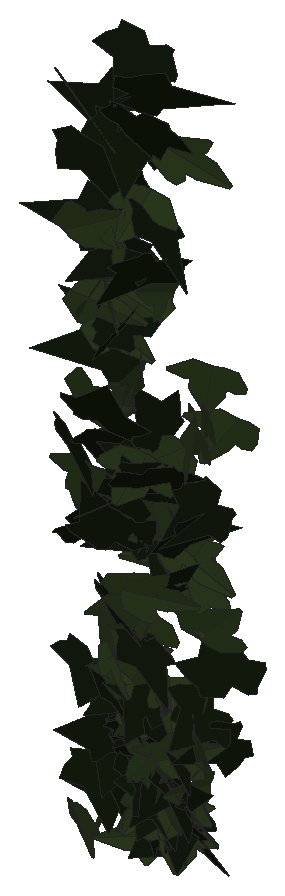
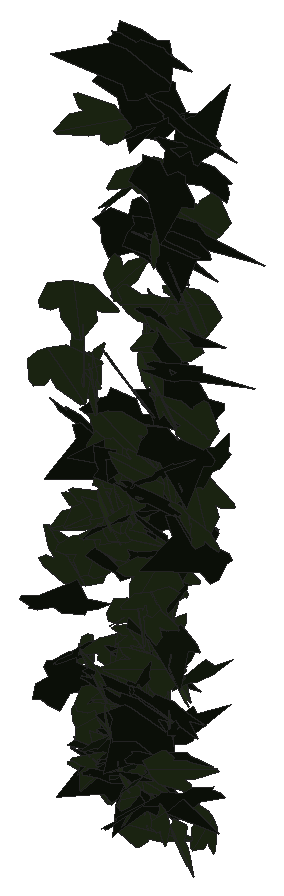
# SketchUp Ruby script. Lengths in inches.
U = 1.inch
M = Sketchup.active_model
def pt(a) = Geom::Point3d.new(a.map { |v| v * U })
def face(e, loops, mat)
  f = e.add_face(loops[0].map { |a| pt(a) })
  loops[1..].each { |l| e.add_face(l.map { |a| pt(a) }).erase! }
  f.material = f.back_material = mat if mat
  f
end
# faces: each face lists its corners as indices into pts; further lists are holes
def faces(e, pts, list, mat = nil) = list.each { |f| face(e, (f[0].is_a?(Array) ? f : [f]).map { |l| l.map { |i| pts[i] } }, mat) }
# xy, xz, yz: faces in a plane at the given z, y or x. An outline is a flat list of corners, or four numbers for a rectangle; further outlines are holes
def ring(l) = l.size == 4 ? [[l[0], l[1]], [l[2], l[1]], [l[2], l[3]], [l[0], l[3]]] : l.each_slice(2).to_a
def flat(e, list, mat, &to3) = list.each { |f| face(e, (f[0].is_a?(Array) ? f : [f]).map { |l| ring(l).map { |u, v| to3.(u, v) } }, mat) }
def xy(e, z, list, mat = nil) = flat(e, list, mat) { |x, y| [x, y, z] }
def xz(e, y, list, mat = nil) = flat(e, list, mat) { |x, z| [x, y, z] }
def yz(e, x, list, mat = nil) = flat(e, list, mat) { |y, z| [x, y, z] }
def lines(e, pts, list) = list.each { |a, b| e.add_line(pt(pts[a]), pt(pts[b])) }
# prism: a flat outline (further loops are holes) pulled along v
def prism(e, loops, v, mat = nil)
  f = face(e, loops, mat); d = Geom::Vector3d.new(v.map { |x| x * U })
  f.pushpull(f.normal.samedirection?(d) ? d.length : -d.length)
end
def box(e, o, s, mat = nil) = prism(e, [[o, [o[0] + s[0], o[1], o[2]], [o[0] + s[0], o[1] + s[1], o[2]], [o[0], o[1] + s[1], o[2]]]], [0, 0, s[2]], mat)
def at(x, y, z, deg = 0) = Geom::Transformation.translation(pt([x, y, z])) * Geom::Transformation.rotation(ORIGIN, Z_AXIS, deg.degrees)
def axes(o, x, y, z) = Geom::Transformation.new([*x, 0, *y, 0, *z, 0, *pt(o).to_a, 1])
def part(name) = M.definitions.add(name)
# library, detail: a bought-in or finely detailed component or shape, given as its bounding box
def library(name, o, s) = part(name).tap { |d| box(d.entities, o, s) }
def detail(e, o, s) = box(e.add_group.entities, o, s)
def put(e, d, t, mat = nil) = e.add_instance(d, t).tap { |i| i.material = mat if mat }
def group(e, t, mat = nil) = e.add_group.tap { |g| g.transformation = t; g.material = mat if mat }.entities
root = M.entities
M.materials.add("1026 AP 7946 SUNNY SIDE UP").color = [254, 231, 186]
M.materials.add("efeu1").color = [18, 25, 13]
M.materials.add("efeu2").color = [43, 57, 29]
c1 = part("ivyleaf_9")
p = [[1.54,2.16,1.25],[1.36,2.04,1.19],[-0.21,0.99,0.68],[-0.71,1.11,0.82],[-0.85,0.86,0.67],[-0.8,0.17,0.21],
  [-0.9,-0.01,0.1],[-0.67,-0.16,-0.02],[-0.08,-0.08,-0.05],[-0.03,-0.6,-0.4],[0.65,-0.88,-0.66],[0.83,-0.6,-0.49],
  [1.29,-0.42,-0.43],[1.8125,-0.07,-0.26],[1.21,0.44,0.15]]
faces(c1.entities,p,[[0,1,2,3,4,5,6,7,8,9,10,11,12,13,14]],"efeu1")
c2 = part("ivyleaf_10")
p = [[0,0.5,-0.03],[-0.0625,2.02,-0.43],[-0.19,2.01,-0.46],[-0.54,1.05,-0.29],[-0.52,0.625,-0.18],[-0.83,0.76,-0.28],
  [-1.16,0.64,-0.33],[-1.15,0.33,-0.24],[-0.77,-0.39,0.02],[-0.3,-0.51,0.16],[0.04,-0.48,0.23],[-0.02,2.01,-0.4375],
  [-0.06,2.01,-0.43],[0.04,-0.49,0.23],[0.67,-0.49,0.14],[1.38,0.36,-0.2],[1.375,0.51,-0.24],[0.81,0.65,-0.19],
  [0.62,0.59,-0.15],[0.6,1.09,-0.28],[0.5,1.23,-0.31]]
faces(c2.entities,p,[[0,1,2,3,4,5,6,7,8,9,10],[11,12,0,13,14,15,16,17,18,19,20]],"efeu2")
put(root,c1,axes([98.49,212.05,269.27],[-0.08526,-0.04089,0.25028],[-0.26767,-0.17357,-0.07103],[0.3023,-0.16522,0.00769]),"1026 AP 7946 SUNNY SIDE UP")
put(root,c1,axes([100.3125,211.96,273.27],[-0.47462,0.04512,-0.05872],[0.08454,-0.03757,-0.30217],[-0.08703,-0.28255,0.02669]),"1026 AP 7946 SUNNY SIDE UP")
put(root,c2,axes([98.93,211.88,271.4375],[-0.2486,-0.25286,-0.0266],[0.04267,0.01175,-0.30667],[0.39716,-0.15954,0.01629]),"1026 AP 7946 SUNNY SIDE UP")
put(root,c1,axes([99.36,211.9375,276.48],[-0.04328,0.20351,-0.24683],[-0.03325,-0.23459,-0.22015],[-0.52438,-0.00192,0.03433]),"1026 AP 7946 SUNNY SIDE UP")
put(root,c2,axes([99.89,212.03,274.12],[0.10442,-0.20831,0.1915],[0.18187,-0.15468,-0.22064],[0.40092,0.12442,0.05022]),"1026 AP 7946 SUNNY SIDE UP")
put(root,c2,axes([99.3,211.71,271.73],[0.1188,0.01973,0.29825],[0.22158,0.2513,-0.0507],[-0.41863,0.13861,0.0578]),"1026 AP 7946 SUNNY SIDE UP")
put(root,c1,axes([98.45,211.95,273.89],[0.44562,-0.02701,0.07349],[-0.11047,0.03739,0.28126],[-0.06013,-0.26883,0.02787]),"1026 AP 7946 SUNNY SIDE UP")
put(root,c1,axes([99.13,211.98,270.85],[0.05244,-0.25972,-0.0269],[0.02039,0.02328,-0.27925],[0.44195,0.02974,0.01607]),"1026 AP 7946 SUNNY SIDE UP")
put(root,c1,axes([97.94,212.08,273.33],[0.07608,-0.21092,0.18856],[0.05391,-0.17609,-0.23326],[0.46636,0.05477,-0.0038]),"1026 AP 7946 SUNNY SIDE UP")
put(root,c2,axes([98.71,211.83,271.2],[-0.01528,0.28786,0.0357],[-0.0625,0.02823,-0.30555],[-0.48723,-0.01265,0.03807]),"1026 AP 7946 SUNNY SIDE UP")
put(root,c1,axes([98.55,211.97,270.13],[0.21081,-0.23004,0.01294],[-0.00284,-0.01803,-0.27991],[0.39132,0.12379,-0.009]),"1026 AP 7946 SUNNY SIDE UP")
put(root,c2,axes([99.02,211.97,270.36],[-0.31309,-0.16797,0.12113],[-0.10904,-0.0997,-0.26681],[0.32824,-0.19334,0.0269]),"1026 AP 7946 SUNNY SIDE UP")
put(root,c2,axes([98.27,211.8,276.67],[-0.19468,-0.13502,0.25878],[0.27493,0.18184,0.19216],[-0.38443,0.19842,0.00638]),"1026 AP 7946 SUNNY SIDE UP")
put(root,c1,axes([99.54,212,269.01],[-0.39901,-0.00249,-0.0961],[0.15113,-0.03869,-0.24905],[-0.01952,-0.2486,0.03617]),"1026 AP 7946 SUNNY SIDE UP")
put(root,c2,axes([98.78,211.89,270.68],[0.12003,0.27677,0.00795],[0.02085,0.0008,-0.30555],[-0.46941,0.0708,-0.01154]),"1026 AP 7946 SUNNY SIDE UP")
put(root,c1,axes([98.2,212.13,270.18],[-0.14201,-0.2201,0.15342],[0.0431,-0.1654,-0.23372],[0.41674,-0.0579,0.07645]),"1026 AP 7946 SUNNY SIDE UP")
put(root,c1,axes([99.3125,212.05,270.1875],[-0.33829,-0.16192,-0.01215],[0.02958,-0.00682,-0.27444],[0.27371,-0.19938,0.01464]),"1026 AP 7946 SUNNY SIDE UP")
put(root,c2,axes([99.08,211.98,273.4375],[0.45671,0.01173,-0.07246],[-0.10874,-0.02673,-0.29867],[-0.02776,0.29767,-0.0222]),"1026 AP 7946 SUNNY SIDE UP")
put(root,c1,axes([99.35,211.76,273.47],[0.33646,0.22451,0.00758],[0.00453,0.00318,-0.32058],[-0.38116,0.19822,0.00287]),"1026 AP 7946 SUNNY SIDE UP")
put(root,c1,axes([99.52,212.02,268.78],[0.01263,0.02538,0.27384],[0.21354,-0.22314,0.0167],[0.37988,0.12459,-0.01849]),"1026 AP 7946 SUNNY SIDE UP")
put(root,c1,axes([99.57,212.11,268.89],[0.01837,-0.23873,0.13227],[0.04929,-0.12501,-0.25663],[0.4561,0.02313,0.0224]),"1026 AP 7946 SUNNY SIDE UP")
put(root,c2,axes([99.14,212.03,277.28],[0.27821,0.18123,-0.16405],[-0.15931,-0.12467,-0.26303],[-0.37287,0.18849,-0.01002]),"1026 AP 7946 SUNNY SIDE UP")
put(root,c2,axes([99.23,211.9375,269.24],[0.26332,-0.18194,-0.08992],[-0.10371,0.05507,-0.25496],[0.32223,0.1664,-0.00858]),"1026 AP 7946 SUNNY SIDE UP")
put(root,c2,axes([99.97,212.16,268.96],[-0.03352,-0.02334,-0.29645],[-0.17499,-0.26543,0.02913],[-0.41865,0.11282,0.01156]),"1026 AP 7946 SUNNY SIDE UP")
put(root,c1,axes([98.6875,211.99,272.21],[0.28824,0.02675,0.2393],[-0.36625,0.04462,0.18444],[-0.02952,-0.2924,0.04828]),"1026 AP 7946 SUNNY SIDE UP")
put(root,c2,axes([99.37,212.02,268.76],[-0.19495,0.11913,-0.18588],[0.18776,-0.13624,-0.17871],[-0.30673,-0.15911,0.00875]),"1026 AP 7946 SUNNY SIDE UP")
put(root,c2,axes([98.11,211.96,268.04],[-0.29628,0.16092,-0.07796],[0.06673,-0.06741,-0.25401],[-0.29383,-0.17757,0.02092]),"1026 AP 7946 SUNNY SIDE UP")
put(root,c1,axes([98.77,212.11,278.14],[-0.13359,-0.27269,0.00935],[0.00737,-0.01404,-0.30392],[0.46331,-0.0784,0.00753]),"1026 AP 7946 SUNNY SIDE UP")
put(root,c1,axes([98.75,211.8,272.84],[0.02401,0.27249,0.04118],[-0.06208,0.03651,-0.28875],[-0.4622,0.00925,0.04092]),"1026 AP 7946 SUNNY SIDE UP")
put(root,c1,axes([98.54,211.96,271.42],[0.33692,-0.191,-0.08782],[-0.1101,0.04723,-0.29401],[0.33351,0.20854,-0.00835]),"1026 AP 7946 SUNNY SIDE UP")
put(root,c2,axes([100.11,211.86,269.88],[-0.24734,0.19341,0.15786],[-0.20793,0.08679,-0.25463],[-0.35368,-0.18628,0.0393]),"1026 AP 7946 SUNNY SIDE UP")
put(root,c2,axes([99.74,211.82,269.4375],[-0.10782,-0.08442,0.26473],[0.17577,0.22674,0.11402],[-0.40917,0.11965,-0.02078]),"1026 AP 7946 SUNNY SIDE UP")
put(root,c2,axes([99.53,212.11,269.21],[0.08542,-0.22565,0.13653],[0.0635,-0.12783,-0.23971],[0.40759,0.0672,0.00873]),"1026 AP 7946 SUNNY SIDE UP")
put(root,c2,axes([99.66,212.03,268.72],[0.42575,0.02925,-0.03108],[-0.04494,-0.02593,-0.26961],[-0.05421,0.25119,-0.02062]),"1026 AP 7946 SUNNY SIDE UP")
put(root,c1,axes([99.11,211.9,278.52],[0.44169,0.07275,-0.14611],[-0.21125,-0.06319,-0.28894],[-0.15825,0.28739,-0.02208]),"1026 AP 7946 SUNNY SIDE UP")
put(root,c1,axes([99.44,212.12,269.72],[0.07739,-0.27307,0.04078],[0.00434,-0.04179,-0.29694],[0.46889,0.04546,-0.00398]),"1026 AP 7946 SUNNY SIDE UP")
put(root,c1,axes([99.54,212.0625,268.88],[0.28147,-0.18304,0.0415],[0.02674,-0.04115,-0.26444],[0.31735,0.16581,-0.01453]),"1026 AP 7946 SUNNY SIDE UP")
put(root,c1,axes([99.9,211.75,272.81],[-0.06446,0.12816,-0.2886],[-0.07842,0.27686,0.13926],[0.47906,0.06257,-0.01603]),"1026 AP 7946 SUNNY SIDE UP")
put(root,c2,axes([99.67,212.03,269.39],[-0.3948,-0.1276,0.05685],[-0.06168,-0.04718,-0.28355],[0.22751,-0.23423,0.02177]),"1026 AP 7946 SUNNY SIDE UP")
put(root,c1,axes([99.21,212.1,277.07],[0.14985,-0.28792,-0.01824],[-0.02233,0.00986,-0.32209],[0.48876,0.08872,-0.00912]),"1026 AP 7946 SUNNY SIDE UP")
put(root,c1,axes([99.11,212.13,270.1875],[-0.41299,-0.06368,0.05582],[-0.07815,-0.03269,-0.26887],[0.1169,-0.24683,0.01747]),"1026 AP 7946 SUNNY SIDE UP")
put(root,c2,axes([99.14,211.9,274.875],[0.11185,-0.22747,-0.19349],[-0.00979,0.19069,-0.2409],[0.46244,0.05905,0.0417]),"1026 AP 7946 SUNNY SIDE UP")
put(root,c1,axes([99.29,212.1875,268.67],[-0.24745,-0.19467,0.04233],[0.01274,-0.05747,-0.25764],[0.33785,-0.14041,0.04072]),"1026 AP 7946 SUNNY SIDE UP")
put(root,c1,axes([98.16,212.09,277.78],[-0.18749,-0.08809,-0.27062],[0.41068,0.08134,-0.14303],[0.19018,-0.26249,0.04207]),"1026 AP 7946 SUNNY SIDE UP")
put(root,c2,axes([98.23,211.97,275.6],[-0.18093,-0.06005,-0.26458],[0.41406,0.04874,-0.12502],[0.11762,-0.26396,0.03311]),"1026 AP 7946 SUNNY SIDE UP")
put(root,c2,axes([99.35,212.01,270.26],[-0.19379,0.23095,-0.0201],[-0.00312,-0.02518,-0.27582],[-0.39377,-0.11346,0.01208]),"1026 AP 7946 SUNNY SIDE UP")
put(root,c2,axes([99.6,212.0625,268.3125],[0.43887,0.08135,0.03336],[0.06002,-0.01243,-0.28934],[-0.13446,0.25998,-0.02028]),"1026 AP 7946 SUNNY SIDE UP")
put(root,c1,axes([98.84,212.14,276.41],[-0.44653,-0.01259,0.02582],[-0.0384,-0.03178,-0.28048],[0.0261,-0.26224,0.02903]),"1026 AP 7946 SUNNY SIDE UP")
put(root,c2,axes([98.94,212.08,270.25],[0.41497,0.08216,-0.01405],[-0.00863,-0.02919,-0.27509],[-0.14127,0.24312,-0.02445]),"1026 AP 7946 SUNNY SIDE UP")
put(root,c2,axes([100.2,212.06,275.12],[-0.41251,-0.12101,0.03925],[-0.03233,-0.04737,-0.29582],[0.19717,-0.26093,0.0336]),"1026 AP 7946 SUNNY SIDE UP")
put(root,c1,axes([99.22,212.09,272.78],[0.24643,0.08014,0.23446],[-0.38294,-0.01237,0.16555],[0.09361,-0.26159,0.06]),"1026 AP 7946 SUNNY SIDE UP")
put(root,c1,axes([99.64,212.01,268.89],[0.34698,-0.11678,-0.10798],[-0.16976,0.02394,-0.25008],[0.19728,0.226,-0.02528]),"1026 AP 7946 SUNNY SIDE UP")
put(root,c2,axes([99.53,212.07,270.28],[0.18975,0.24659,-0.05557],[-0.00721,-0.05843,-0.28989],[-0.42887,0.11008,-0.01971]),"1026 AP 7946 SUNNY SIDE UP")
put(root,c1,axes([99.22,212.02,271.58],[0.31537,0.19631,0.03215],[-0.05859,-0.00504,0.28837],[0.33135,-0.18773,0.02039]),"1026 AP 7946 SUNNY SIDE UP")
put(root,c2,axes([98.67,212.2,276.57],[-0.00223,-0.25766,0.16923],[0.1735,-0.15504,-0.24825],[0.44939,0.05858,0.09668]),"1026 AP 7946 SUNNY SIDE UP")
put(root,c1,axes([98.96,211.9,273.22],[0.07735,0.05221,-0.30263],[0.16453,0.26738,0.07316],[0.46061,-0.10428,0.02469]),"1026 AP 7946 SUNNY SIDE UP")
put(root,c1,axes([99.32,212.13,268.66],[0.02556,-0.26391,-0.0804],[-0.01808,0.07115,-0.28192],[0.46387,0.01731,-0.00656]),"1026 AP 7946 SUNNY SIDE UP")
put(root,c2,axes([98.25,212.0625,272.97],[-0.47545,0.00098,0.09994],[-0.15759,-0.03354,-0.29834],[0.01643,-0.29331,0.0303]),"1026 AP 7946 SUNNY SIDE UP")
put(root,c1,axes([98.87,211.91,270.69],[0.02386,0.28264,0.04639],[-0.07026,0.0413,-0.29887],[-0.47937,0.00801,0.04612]),"1026 AP 7946 SUNNY SIDE UP")
put(root,c1,axes([99.98,212.31,270.03],[-0.19514,-0.20612,0.16734],[-0.10483,-0.15036,-0.24812],[0.40028,-0.13986,0.0166]),"1026 AP 7946 SUNNY SIDE UP")
put(root,c2,axes([98.52,212.09,275.77],[-0.08664,0.25394,-0.05518],[0.00645,-0.05516,-0.27797],[-0.44097,-0.0507,0.00677]),"1026 AP 7946 SUNNY SIDE UP")
put(root,c1,axes([98.48,212.09,276.67],[-0.30459,0.08576,0.20225],[-0.31719,0.03835,-0.20934],[-0.14904,-0.25689,0.0322]),"1026 AP 7946 SUNNY SIDE UP")
put(root,c1,axes([98.15,212.19,278.04],[0.24113,-0.26065,0.08242],[-0.03504,0.08011,0.31822],[-0.4617,-0.14221,0.0189]),"1026 AP 7946 SUNNY SIDE UP")
put(root,c2,axes([98.21,212.11,275.38],[-0.04328,-0.26983,0.00694],[0.01798,0.00904,0.2901],[-0.458,0.02585,0.01073]),"1026 AP 7946 SUNNY SIDE UP")
put(root,c1,axes([99.57,212.24,268.47],[-0.30472,-0.11647,-0.17771],[0.32615,-0.03237,-0.2004],[0.10334,-0.2413,0.10845]),"1026 AP 7946 SUNNY SIDE UP")
put(root,c2,axes([98.39,212.23,270.24],[0.19197,-0.19946,0.14498],[0.09895,-0.12548,-0.24701],[0.39969,0.12687,-0.00849]),"1026 AP 7946 SUNNY SIDE UP")
put(root,c1,axes([98.45,212.1,274.88],[0.10949,0.22576,0.13438],[-0.08997,-0.11197,0.24907],[0.42671,-0.08154,0.01804]),"1026 AP 7946 SUNNY SIDE UP")
put(root,c1,axes([99,211.96,278.8125],[0.29194,0.0355,0.27226],[0.41689,0.06472,-0.18691],[-0.12461,0.29971,0.01255]),"1026 AP 7946 SUNNY SIDE UP")
put(root,c1,axes([99.54,212.11,268.41],[0.42207,-0.08576,-0.0056],[-0.0199,-0.02142,-0.28069],[0.14438,0.24774,-0.0223]),"1026 AP 7946 SUNNY SIDE UP")
put(root,c2,axes([99.23,212.11,272.77],[-0.39394,-0.12203,-0.03602],[0.05942,0.00055,-0.28661],[0.19023,-0.25287,0.01494]),"1026 AP 7946 SUNNY SIDE UP")
put(root,c2,axes([99.16,212.3,268.72],[0.05841,-0.19152,0.2037],[0.10486,-0.18844,-0.20094],[0.42122,0.07347,0.02178]),"1026 AP 7946 SUNNY SIDE UP")
put(root,c2,axes([98.9,212.2,274.65],[0.05826,-0.25237,0.04869],[0.00076,-0.04915,-0.27328],[0.43634,0.03378,-0.00603]),"1026 AP 7946 SUNNY SIDE UP")
put(root,c2,axes([98.7,212.02,269.875],[-0.1634,0.15587,0.17613],[-0.20804,0.11197,-0.19116],[-0.32065,-0.15208,0.03427]),"1026 AP 7946 SUNNY SIDE UP")
put(root,c1,axes([99.46,211.94,274.0625],[-0.0546,0.16525,0.26263],[-0.1632,0.23371,-0.1699],[-0.44765,-0.10536,0.02991]),"1026 AP 7946 SUNNY SIDE UP")
put(root,c1,axes([98.63,212.08,276.54],[0.30356,0.11456,-0.17944],[-0.23576,-0.0966,-0.22864],[-0.25423,0.22637,-0.00222]),"1026 AP 7946 SUNNY SIDE UP")
put(root,c2,axes([98.96,212.05,270.56],[0.16664,0.19262,0.15119],[0.12001,0.11956,-0.22965],[-0.38465,0.12075,-0.00615]),"1026 AP 7946 SUNNY SIDE UP")
put(root,c2,axes([99.12,212.15,270.1875],[-0.40072,0.09197,0.04885],[-0.10835,-0.04549,-0.2629],[-0.13536,-0.23585,0.06583]),"1026 AP 7946 SUNNY SIDE UP")
put(root,c2,axes([98.99,212.27,268.38],[0.13723,0.14304,-0.19504],[-0.17313,-0.15346,-0.17779],[-0.35581,0.12984,0.01128]),"1026 AP 7946 SUNNY SIDE UP")
put(root,c2,axes([98.95,212.26,268.4],[0.16258,0.16533,-0.16092],[-0.1066,-0.13946,-0.20608],[-0.36658,0.11388,-0.01144]),"1026 AP 7946 SUNNY SIDE UP")
put(root,c2,axes([98.96,212.17,269.22],[-0.42744,-0.02083,0.07272],[0.11088,0.03298,0.26945],[-0.04853,0.25878,-0.02479]),"1026 AP 7946 SUNNY SIDE UP")
put(root,c2,axes([100.09,212.07,274.53],[-0.23764,0.20492,0.14312],[-0.19822,0.07485,-0.25674],[-0.33385,-0.19031,0.05056]),"1026 AP 7946 SUNNY SIDE UP")
put(root,c2,axes([99.36,212.17,273.27],[-0.43994,-0.01915,0.04062],[-0.05752,-0.03955,-0.28667],[0.03824,-0.27979,0.03606]),"1026 AP 7946 SUNNY SIDE UP")
put(root,c2,axes([98.8125,212.14,271.57],[-0.35546,-0.10517,-0.09093],[0.14305,0.01768,-0.24963],[0.17757,-0.22476,0.01907]),"1026 AP 7946 SUNNY SIDE UP")
put(root,c1,axes([99.3,212.05,267.97],[0.04411,-0.02278,0.26282],[-0.10737,0.23829,0.03413],[-0.40504,-0.06565,0.01958]),"1026 AP 7946 SUNNY SIDE UP")
put(root,c2,axes([98.67,212.19,273.18],[-0.38397,0.15901,0.03637],[-0.1385,-0.06427,-0.27734],[-0.23792,-0.2192,0.10276]),"1026 AP 7946 SUNNY SIDE UP")
put(root,c2,axes([98,212.21,273.94],[-0.17344,0.00845,0.27623],[0.43778,0.01307,0.1091],[-0.01537,0.2771,-0.00969]),"1026 AP 7946 SUNNY SIDE UP")
put(root,c1,axes([98.95,212.3,279.32],[-0.42491,-0.08185,-0.08873],[0.14267,0.00547,-0.28105],[0.13507,-0.26328,0.01771]),"1026 AP 7946 SUNNY SIDE UP")
put(root,c2,axes([99.95,212.09,274.18],[-0.26267,0.1698,0.1675],[-0.23423,0.07637,-0.2408],[-0.28463,-0.21954,0.04358]),"1026 AP 7946 SUNNY SIDE UP")
put(root,c1,axes([98.91,212.37,270.03],[-0.03265,-0.05735,0.24903],[0.03995,-0.23343,-0.06259],[0.40596,0.01836,0.02619]),"1026 AP 7946 SUNNY SIDE UP")
put(root,c2,axes([98.97,212.3,267.85],[0.12192,0.00357,-0.24605],[-0.35232,-0.10259,-0.07256],[-0.16788,0.21789,-0.02641]),"1026 AP 7946 SUNNY SIDE UP")
put(root,c2,axes([99.58,212.125,268.5],[0.16603,0.21283,0.11649],[0.10436,0.08813,-0.24884],[-0.38993,0.11421,-0.017]),"1026 AP 7946 SUNNY SIDE UP")
put(root,c1,axes([99.1,212.25,268.8125],[0.26415,-0.18729,0.04655],[0.08053,-0.02002,-0.25977],[0.31728,0.16101,0.02718]),"1026 AP 7946 SUNNY SIDE UP")
put(root,c1,axes([98.99,212.25,272.32],[-0.38519,0.09361,0.03807],[-0.07129,-0.01231,-0.26134],[-0.15351,-0.22916,0.02585]),"1026 AP 7946 SUNNY SIDE UP")
put(root,c1,axes([98.875,212.22,268.43],[-0.11281,0.00389,-0.26879],[-0.38799,-0.10861,0.06144],[-0.17673,0.23597,0.0367]),"1026 AP 7946 SUNNY SIDE UP")
put(root,c1,axes([98,212.03,272.17],[0.27391,0.14899,0.18303],[0.24319,0.09261,-0.23253],[-0.2952,0.21454,-0.02173]),"1026 AP 7946 SUNNY SIDE UP")
put(root,c2,axes([98.92,212.14,269.71],[0.15026,0.08253,0.253],[0.33257,0.13135,-0.12642],[-0.26172,0.21429,-0.01539]),"1026 AP 7946 SUNNY SIDE UP")
put(root,c1,axes([100.26,212.44,269.64],[-0.08847,-0.06742,-0.26859],[0.09099,-0.26277,0.05569],[-0.41295,-0.04345,0.06981]),"1026 AP 7946 SUNNY SIDE UP")
put(root,c1,axes([98.78,212.18,275.17],[-0.11859,0.10059,0.25021],[-0.36171,0.10694,-0.11663],[-0.23232,-0.21785,0.05387]),"1026 AP 7946 SUNNY SIDE UP")
put(root,c1,axes([99.17,212.43,267.93],[-0.16818,-0.1416,0.17778],[-0.10889,-0.15752,-0.18493],[0.35661,-0.11488,0.02738]),"1026 AP 7946 SUNNY SIDE UP")
put(root,c1,axes([98.21,212.34,268.59],[-0.1389,-0.25209,-0.07059],[0.04143,0.06185,-0.27479],[0.40809,-0.09208,0.00387]),"1026 AP 7946 SUNNY SIDE UP")
put(root,c1,axes([98.75,212.4,268.73],[0.02971,-0.24978,0.08462],[0.01307,-0.08317,-0.25853],[0.41394,0.02055,0.00209]),"1026 AP 7946 SUNNY SIDE UP")
put(root,c2,axes([99.2,212.43,275.79],[-0.05226,-0.07479,-0.26571],[-0.15187,-0.23046,0.08336],[-0.4113,0.0946,0.00298]),"1026 AP 7946 SUNNY SIDE UP")
put(root,c1,axes([98.56,212.16,278.33],[-0.22742,0.14869,0.20285],[-0.25248,0.11665,-0.21114],[-0.31829,-0.19877,0.02255]),"1026 AP 7946 SUNNY SIDE UP")
put(root,c1,axes([98.98,212.19,268.43],[0.40217,-0.0539,-0.12581],[-0.20256,-0.00057,-0.25882],[0.08163,0.26415,-0.02239]),"1026 AP 7946 SUNNY SIDE UP")
put(root,c1,axes([98.5,212.38,274.74],[-0.39094,0.00094,0.18538],[-0.27903,-0.09178,-0.2348],[0.09241,-0.27312,0.0753]),"1026 AP 7946 SUNNY SIDE UP")
put(root,c2,axes([99.99,212.23,271.18],[-0.38583,-0.06835,0.14576],[0.20126,0.06647,0.26143],[-0.14426,0.27553,-0.02511]),"1026 AP 7946 SUNNY SIDE UP")
put(root,c2,axes([99.64,212.31,271.6875],[-0.43755,-0.10065,-0.04351],[0.13154,-0.10125,-0.26769],[0.12786,-0.24028,0.12648]),"1026 AP 7946 SUNNY SIDE UP")
put(root,c2,axes([98.34,212.18,275.13],[0.20342,0.09152,0.23278],[0.32311,0.10431,-0.15873],[-0.23343,0.22414,-0.01685]),"1026 AP 7946 SUNNY SIDE UP")
put(root,c2,axes([98.98,212.27,270.99],[-0.43322,-0.02522,0.06308],[-0.0865,-0.06897,-0.26736],[0.06683,-0.25275,0.06284]),"1026 AP 7946 SUNNY SIDE UP")
put(root,c1,axes([98.41,212.16,273.6],[0.13483,0.23646,-0.07195],[-0.03586,-0.06705,-0.26798],[-0.41722,0.08218,-0.00022]),"1026 AP 7946 SUNNY SIDE UP")
put(root,c2,axes([99.38,212.28,273.61],[0.36263,-0.04286,-0.18137],[-0.28413,0.02358,-0.23278],[0.08199,0.27127,-0.00452]),"1026 AP 7946 SUNNY SIDE UP")
put(root,c2,axes([98.76,212.32,273.04],[-0.00344,-0.02062,-0.2807],[0.40137,-0.11437,0.00608],[-0.1945,-0.23565,0.01752]),"1026 AP 7946 SUNNY SIDE UP")
put(root,c2,axes([100.27,212.36,274.25],[-0.33215,-0.16514,0.14756],[-0.1184,-0.13338,-0.27182],[0.32372,-0.21822,0.05198]),"1026 AP 7946 SUNNY SIDE UP")
put(root,c1,axes([99.6,212.32,269.77],[-0.37624,0.0542,0.11932],[-0.19204,0.0012,-0.243],[-0.08323,-0.24777,0.0213]),"1026 AP 7946 SUNNY SIDE UP")
put(root,c1,axes([98.9,212.17,269.22],[0.38924,0.10232,-0.0019],[0.00973,-0.02044,-0.26816],[-0.1735,0.22841,-0.01929]),"1026 AP 7946 SUNNY SIDE UP")
put(root,c1,axes([98.92,212.29,269.48],[0.05165,0.17097,-0.18274],[-0.06909,-0.16823,-0.18808],[-0.40697,0.05026,0.00874]),"1026 AP 7946 SUNNY SIDE UP")
put(root,c2,axes([99.33,212.41,272.01],[-0.06653,0.00578,0.26452],[-0.24831,-0.20209,-0.02261],[0.338,-0.14733,0.03546]),"1026 AP 7946 SUNNY SIDE UP")
put(root,c2,axes([99.21,212.45,272.23],[-0.0396,0.06082,0.24829],[-0.0639,-0.23027,0.05759],[0.40065,-0.03072,0.03372]),"1026 AP 7946 SUNNY SIDE UP")
put(root,c2,axes([98.67,212.34,271.33],[0.26994,0.16558,-0.09038],[-0.08124,-0.0738,-0.24624],[-0.30661,0.16534,-0.01432]),"1026 AP 7946 SUNNY SIDE UP")
put(root,c1,axes([98.52,212.42,269.07],[-0.31728,-0.18628,-0.03144],[0.04696,0.01036,-0.28206],[0.31603,-0.18855,0.01035]),"1026 AP 7946 SUNNY SIDE UP")
put(root,c2,axes([99.16,212.23,268.5625],[0.03847,-0.02827,-0.26047],[-0.36088,0.11833,-0.03432],[0.20524,0.21337,-0.01153]),"1026 AP 7946 SUNNY SIDE UP")
put(root,c1,axes([99.22,212.48,272.27],[-0.15107,-0.27143,0.05995],[-0.02352,-0.05806,-0.29692],[0.43638,-0.09709,0.00475]),"1026 AP 7946 SUNNY SIDE UP")
put(root,c2,axes([99.46,212.16,272.63],[0.15154,-0.06115,-0.25901],[-0.22229,0.20628,-0.10502],[0.35906,0.15351,0.04429]),"1026 AP 7946 SUNNY SIDE UP")
put(root,c2,axes([98.97,212.34,275.49],[0.17702,0.11752,0.23428],[-0.34356,-0.09462,0.15744],[0.24049,-0.22168,0.05247]),"1026 AP 7946 SUNNY SIDE UP")
put(root,c2,axes([97.99,212.39,272.68],[0.3879,-0.08465,0.10768],[0.14219,-0.06452,-0.25993],[0.17386,0.24164,-0.02766]),"1026 AP 7946 SUNNY SIDE UP")
put(root,c1,axes([98.16,212.46,276.08],[-0.20027,0.00119,-0.25557],[0.37261,-0.1042,-0.11813],[-0.1594,-0.24506,0.04495]),"1026 AP 7946 SUNNY SIDE UP")
put(root,c2,axes([98.52,212.41,268.23],[-0.24204,0.11722,-0.17763],[0.13556,-0.156,-0.19188],[-0.31941,-0.15503,0.05317]),"1026 AP 7946 SUNNY SIDE UP")
put(root,c2,axes([98.99,212.21,271.04],[0.12195,-0.15034,-0.19728],[-0.07236,0.17918,-0.17367],[0.39456,0.07933,0.02913]),"1026 AP 7946 SUNNY SIDE UP")
put(root,c2,axes([99.51,212.22,272.31],[0.2013,0.13348,0.20446],[0.20081,0.14787,-0.18895],[-0.33796,0.16736,0.00952]),"1026 AP 7946 SUNNY SIDE UP")
put(root,c2,axes([98.77,212.19,274.27],[-0.0306,0.09985,0.25574],[-0.36285,0.12724,-0.07284],[-0.24437,-0.20144,0.07613]),"1026 AP 7946 SUNNY SIDE UP")
put(root,c1,axes([99.24,212.47,268.59],[-0.3112,-0.1629,-0.02317],[0.08138,-0.0252,-0.25727],[0.26635,-0.18263,0.05154]),"1026 AP 7946 SUNNY SIDE UP")
put(root,c2,axes([99.47,212.22,277.99],[0.19536,0.07819,0.25965],[0.30092,0.16505,-0.14534],[-0.30845,0.21055,0.02266]),"1026 AP 7946 SUNNY SIDE UP")
put(root,c2,axes([99.56,212.26,272.17],[0.22372,0.1231,0.23368],[0.3201,0.11097,-0.18874],[-0.27655,0.22803,-0.02943]),"1026 AP 7946 SUNNY SIDE UP")
put(root,c2,axes([99.42,212.4,272.5],[0.14277,-0.26786,0.03403],[0.00602,-0.03517,-0.29147],[0.42464,0.09056,-0.00731]),"1026 AP 7946 SUNNY SIDE UP")
put(root,c1,axes([98.52,212.52,273.25],[-0.16427,-0.20834,0.10753],[-0.05377,-0.09888,-0.24699],[0.39097,-0.10113,0.01121]),"1026 AP 7946 SUNNY SIDE UP")
put(root,c1,axes([99.08,212.4375,269.73],[-0.42578,-0.02832,-0.0357],[0.05948,-0.01744,-0.26953],[0.04366,-0.25238,0.01904]),"1026 AP 7946 SUNNY SIDE UP")
put(root,c2,axes([98.65,212.34,270.27],[-0.20462,-0.02564,-0.2414],[0.38377,-0.03103,-0.12622],[-0.02629,-0.25349,0.03624]),"1026 AP 7946 SUNNY SIDE UP")
put(root,c1,axes([100.33,212.27,270.58],[-0.4032,-0.10642,0.09846],[0.1201,0.06545,0.28478],[-0.19091,0.26593,-0.02879]),"1026 AP 7946 SUNNY SIDE UP")
put(root,c1,axes([98.94,212.42,272.84],[-0.42046,0.04325,0.08234],[-0.1311,-0.01981,-0.27727],[-0.05601,-0.27832,0.03086]),"1026 AP 7946 SUNNY SIDE UP")
put(root,c2,axes([99.71,212.38,270.05],[0.25543,-0.1972,-0.0248],[-0.04423,0.00596,-0.26485],[0.33366,0.15175,-0.01612]),"1026 AP 7946 SUNNY SIDE UP")
put(root,c1,axes([98.5,212.29,277.51],[0.36616,-0.01221,-0.18979],[-0.30089,-0.0307,-0.22926],[-0.01718,0.2774,-0.0298]),"1026 AP 7946 SUNNY SIDE UP")
put(root,c1,axes([98.53,212.47,269.9375],[-0.43323,-0.04251,-0.07001],[0.11708,-0.02252,-0.2751],[0.06015,-0.26236,0.03118]),"1026 AP 7946 SUNNY SIDE UP")
put(root,c2,axes([98.2,212.43,268.01],[0.17025,-0.23135,0.04363],[0.01591,-0.04362,-0.2704],[0.39939,0.10036,-0.00783]),"1026 AP 7946 SUNNY SIDE UP")
put(root,c2,axes([99.2,212.37,272.16],[0.24905,0.23384,-0.01202],[0.01027,-0.02009,-0.29057],[-0.36812,0.15765,-0.01623]),"1026 AP 7946 SUNNY SIDE UP")
put(root,c2,axes([98.4375,212.45,268.91],[0.06716,0.08776,0.24166],[-0.28223,-0.1549,0.09399],[0.29644,-0.16736,0.03474]),"1026 AP 7946 SUNNY SIDE UP")
